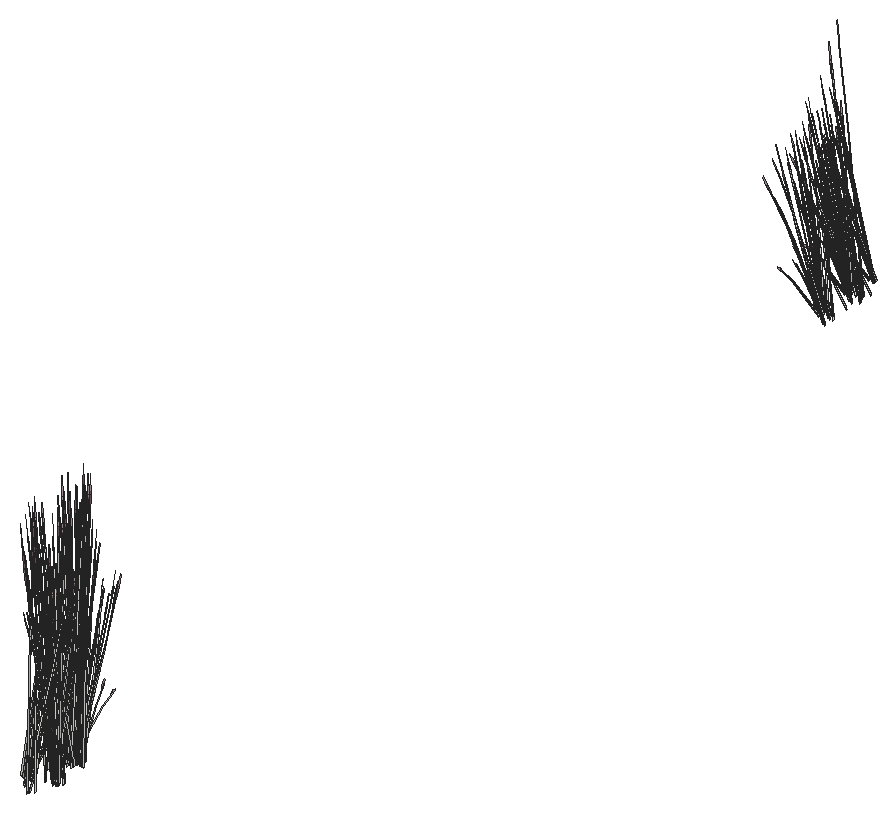
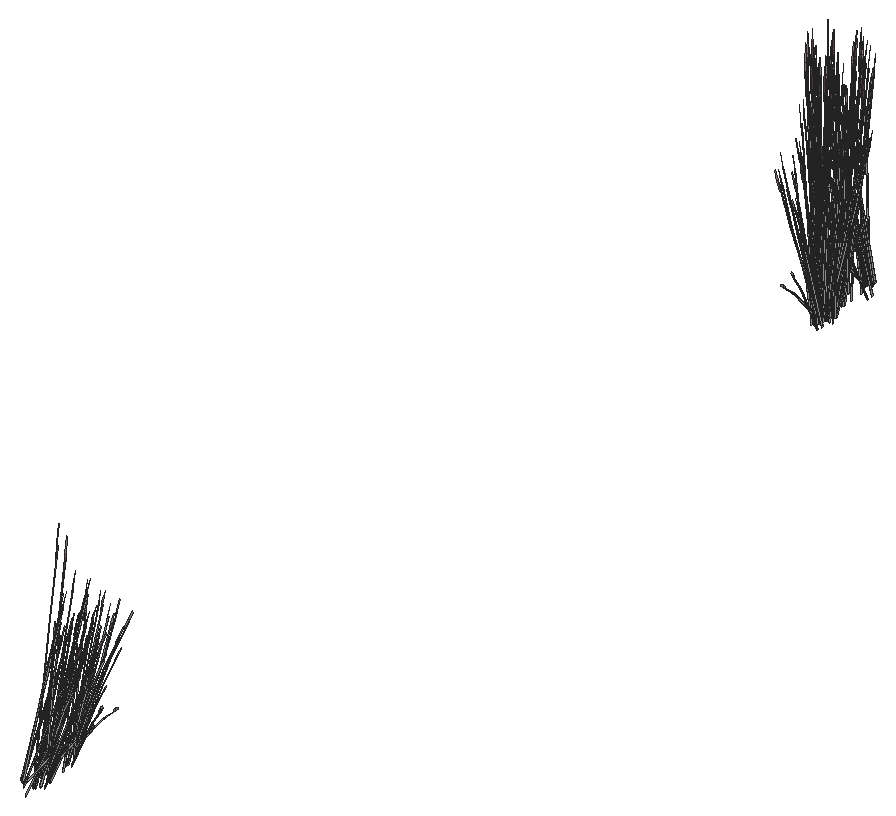
# SketchUp Ruby script. Lengths in inches.
U = 1.inch
M = Sketchup.active_model
def pt(a) = Geom::Point3d.new(a.map { |v| v * U })
def face(e, loops, mat)
  f = e.add_face(loops[0].map { |a| pt(a) })
  loops[1..].each { |l| e.add_face(l.map { |a| pt(a) }).erase! }
  f.material = f.back_material = mat if mat
  f
end
# faces: each face lists its corners as indices into pts; further lists are holes
def faces(e, pts, list, mat = nil) = list.each { |f| face(e, (f[0].is_a?(Array) ? f : [f]).map { |l| l.map { |i| pts[i] } }, mat) }
# xy, xz, yz: faces in a plane at the given z, y or x. An outline is a flat list of corners, or four numbers for a rectangle; further outlines are holes
def ring(l) = l.size == 4 ? [[l[0], l[1]], [l[2], l[1]], [l[2], l[3]], [l[0], l[3]]] : l.each_slice(2).to_a
def flat(e, list, mat, &to3) = list.each { |f| face(e, (f[0].is_a?(Array) ? f : [f]).map { |l| ring(l).map { |u, v| to3.(u, v) } }, mat) }
def xy(e, z, list, mat = nil) = flat(e, list, mat) { |x, y| [x, y, z] }
def xz(e, y, list, mat = nil) = flat(e, list, mat) { |x, z| [x, y, z] }
def yz(e, x, list, mat = nil) = flat(e, list, mat) { |y, z| [x, y, z] }
def lines(e, pts, list) = list.each { |a, b| e.add_line(pt(pts[a]), pt(pts[b])) }
# prism: a flat outline (further loops are holes) pulled along v
def prism(e, loops, v, mat = nil)
  f = face(e, loops, mat); d = Geom::Vector3d.new(v.map { |x| x * U })
  f.pushpull(f.normal.samedirection?(d) ? d.length : -d.length)
end
def box(e, o, s, mat = nil) = prism(e, [[o, [o[0] + s[0], o[1], o[2]], [o[0] + s[0], o[1] + s[1], o[2]], [o[0], o[1] + s[1], o[2]]]], [0, 0, s[2]], mat)
def at(x, y, z, deg = 0) = Geom::Transformation.translation(pt([x, y, z])) * Geom::Transformation.rotation(ORIGIN, Z_AXIS, deg.degrees)
def axes(o, x, y, z) = Geom::Transformation.new([*x, 0, *y, 0, *z, 0, *pt(o).to_a, 1])
def part(name) = M.definitions.add(name)
# library, detail: a bought-in or finely detailed component or shape, given as its bounding box
def library(name, o, s) = part(name).tap { |d| box(d.entities, o, s) }
def detail(e, o, s) = box(e.add_group.entities, o, s)
def put(e, d, t, mat = nil) = e.add_instance(d, t).tap { |i| i.material = mat if mat }
def group(e, t, mat = nil) = e.add_group.tap { |g| g.transformation = t; g.material = mat if mat }.entities
root = M.entities
M.materials.add("LightPink_Translucent").color = [144, 107, 117]
M.materials["LightPink_Translucent"].alpha = 0.75
c1 = part("blade")
p = [[2.15,0.21,22],[0,0.17,0],[0.09,0.45,0],[2.18,0.31,22],[2.29,0.31,22],[0.38,0.45,0],
  [2.48,0.24,33],[2.49,0.24,33],[2.48,0.22,33]]
faces(c1.entities,p,[[0,1,2,3],[4,5,2,3],[6,3,4,7],[8,0,3,6]])
c2 = part("seeds")
p = [[0.3,-0.1,1.38],[-0.01,-0.03,1.59],[-0.01,-0.03,0.03],[0.14,-0.07,-0.07],[0.29,-0.03,3],[0.15,0.01,3.11]]
faces(c2.entities,p,[[0,1,2,3],[1,0,4,5]],"LightPink_Translucent")
c3 = part("blade with seeds")
put(c3.entities,c1,at(0,0,0))
put(c3.entities,c2,axes([2.4,0.25,30.99],[1.5799,-0.05474,1.17369],[-0.12525,1.92788,0.29478],[-0.07173,-0.02425,1.56792]))
put(root,c3,axes([406.86,60.78,-9.79],[0.31974,0.54466,0],[-0.53494,0.30375,-0.48057],[-0.12184,0.06918,1.52448]))
put(root,c3,axes([406.59,58.62,-9.35],[-0.01397,-0.51177,1.31553],[0.63227,0.13266,0.557],[-0.14954,0.28003,1.24175]))
put(root,c3,axes([405.24,60.67,-7.3],[0.15418,-0.41799,0.32977],[0.44981,0.12192,-0.42575],[0.04124,0.16829,0.81462]))
put(root,c3,axes([406.28,64.63,-9.69],[0,0.54355,0.46235],[-0.57217,0,0],[0,-0.1238,1.46668]))
put(root,c3,axes([407.63,65.07,-9.94],[-0.30722,-0.45622,-0.41661],[0.46535,-0.32126,0.2005],[-0.09942,-0.05645,1.33761]))
put(root,c3,axes([407.58,64.91,-9.47],[-0.24813,0.48978,0.41661],[-0.51557,-0.23571,-0.2005],[0,-0.1129,1.33761]))
put(root,c3,axes([405.85,62.16,-6.74],[0.35341,-0.31182,-0.06041],[0.32382,0.34152,-0.27392],[0.0228,0.09677,0.90349]))
put(root,c3,axes([405.1,61.05,-7.6],[-0.37684,0.18473,0.05988],[-0.18445,-0.33686,0.47138],[0.03639,0.14849,0.71878]))
put(root,c3,axes([404.05,60.28,-6.97],[0.56206,0.02693,-0.12569],[-0.01536,0.50991,-0.69765],[-0.03904,0.19638,1.06006]))
put(root,c3,axes([405.09,60.84,-7.3125],[0.50045,-0.25306,-0.11324],[0.24593,0.44915,-0.62851],[0.06603,0.18927,0.95501]))
put(root,c3,axes([405.24,61.01,-7.28],[-0.50393,-0.1421,0.49617],[0.17232,-0.46717,0.40911],[0.03028,0.18372,1.0267]))
put(root,c3,axes([407.75,65.02,-9.8],[0.64638,0.11452,0.42607],[-0.13155,0.64678,0.16719],[-0.09446,-0.06245,1.47927]))
put(root,c3,axes([405.18,60.94,-10.61],[0.08277,-0.02958,1.6421],[0.49786,0.16279,-0.25086],[0.01456,0.18348,0.2797]))
put(root,c3,axes([406.79,66.08,-10.11],[-0.12013,-0.47362,-0.28847],[0.47712,-0.13449,0.28847],[-0.09619,-0.05462,1.29413]))
put(root,c3,axes([404.4375,60.47,-7.34],[0.3661,0.36521,-0.52818],[-0.38674,0.31985,-0.40911],[-0.0557,0.18556,1.01061]))
put(root,c3,axes([404.04,61.02,-9.37],[0.46459,-0.09625,0.0606],[0.10681,0.38778,-0.80367],[-0.02945,0.1963,0.72038]))
put(root,c3,axes([405.52,60.82,-7.64],[0.50273,0.13626,-0.47583],[-0.17232,0.46717,-0.36857],[0.0461,0.18809,0.91046]))
put(root,c3,axes([406.65,66.29,-10.12],[-0.47863,-0.27177,-0.46235],[0.28609,-0.48733,0],[-0.10901,-0.0619,1.46668]))
put(root,c3,axes([405.29,61.11,-7.78],[-0.15418,0.41799,-0.32977],[-0.44981,-0.12192,0.42575],[0.04124,0.16829,0.81462]))
put(root,c3,axes([407.95,65.33,-9.52],[-0.51635,0.36087,-0.27094],[-0.34336,-0.5099,-0.46562],[-0.1274,-0.05178,1.4872]))
put(root,c3,axes([404.85,59.94,-8.39],[-0.01252,-0.20862,1.59586],[0.54251,0.1384,0.12904],[-0.03356,0.2973,0.68222]))
put(root,c3,axes([407.91,65.49,-9.5625],[-0.09866,0.48509,0.13483],[-0.48202,-0.0842,-0.38503],[-0.08772,-0.04981,1.18024]))
put(root,c3,axes([405.34,60.73,-7.36],[0.24409,0.44196,-0.66157],[-0.50245,0.2463,0.07984],[0.05708,0.21354,0.93586]))
put(root,c3,axes([404.97,61.85,-7.61],[0.06483,0.08753,1.62908],[0.52315,0.03439,-0.25764],[0.05261,0.19303,0.13065]))
put(root,c3,axes([408.53,65.49,-9.7],[-0.49938,-0.43748,-0.23459],[0.42021,-0.49126,0.51337],[-0.13447,0.05118,1.56642]))
put(root,c3,axes([407.22,66.33,-9.69],[0.47863,0.27177,0.46235],[-0.28609,0.48733,0],[-0.10901,-0.0619,1.46668]))
put(root,c3,axes([406.94,66.61,-9.79],[-0.31974,0.54466,0],[-0.53494,-0.30375,-0.48057],[-0.12184,-0.06918,1.52448]))
put(root,c3,axes([405.96,70.8125,-7.36],[-0.24409,-0.44196,-0.66157],[0.50245,-0.2463,0.07984],[-0.05708,-0.21354,0.93586]))
put(root,c3,axes([408.28,65.4,-9.94],[-0.55535,0.03355,-0.41661],[-0.05022,-0.55698,0.2005],[-0.09942,0.05645,1.33761]))
put(root,c3,axes([405.54,69.83,-10.61],[-0.08578,0.01958,1.6421],[-0.47437,-0.22044,-0.25086],[0.00796,-0.18387,0.2797]))
put(root,c3,axes([408.9,66.69,-9.96],[-0.31576,-0.54657,-0.04789],[0.53494,-0.30375,0.48057],[-0.13182,0.05204,1.52373]))
put(root,c3,axes([406,70.4375,-7.78],[0.15418,-0.41799,-0.32977],[0.44981,0.12192,0.42575],[-0.04124,-0.16829,0.81462]))
put(root,c3,axes([407.64,70.07,-7.62],[-0.05194,0.04152,1.65179],[-0.50886,-0.14007,-0.15608],[-0.01842,-0.18118,0.29231]))
put(root,c3,axes([405.77,70.73,-7.64],[-0.50273,-0.13626,-0.47583],[0.17232,-0.46717,-0.36857],[-0.0461,-0.18809,0.91046]))
put(root,c3,axes([406.08,69.56,-9.42],[0.06561,0.31695,1.06958],[-0.36394,-0.17555,0.78586],[0.03916,-0.16229,0.23558]))
put(root,c3,axes([408.75,66.62,-10.11],[-0.47712,-0.13449,-0.28847],[0.12013,-0.47362,0.28847],[-0.09619,0.05462,1.29413]))
put(root,c3,axes([406.11,65.29,-7.3],[0.44516,-0.07768,0.32977],[0.11755,0.44407,-0.42575],[-0.12757,0.11927,0.81462]))
put(root,c3,axes([406.06,70.54,-7.59],[0.50393,0.1421,0.447],[-0.17232,0.46717,0.36857],[-0.03028,-0.18372,0.92496]))
put(root,c3,axes([406.2,70.7,-7.3125],[-0.50045,0.25306,-0.11324],[-0.24593,-0.44915,-0.62851],[-0.06603,-0.18927,0.95501]))
put(root,c3,axes([407.24,71.27,-7.3125],[-0.56206,-0.02693,-0.11324],[0.01536,-0.50991,-0.62851],[0.03904,-0.19638,0.95501]))
put(root,c3,axes([406.19,70.5,-7.6],[0.37684,-0.18473,0.05988],[0.18445,0.33686,0.47138],[-0.03639,-0.14849,0.71878]))
put(root,c3,axes([408.67,65.25,-9.52],[0.05959,0.62022,-0.27094],[-0.62068,0.0375,-0.46562],[-0.1093,0.08261,1.4872]))
put(root,c3,axes([405.1,66.55,-6.74],[0.45129,0.14509,-0.06041],[-0.13882,0.44656,-0.27392],[-0.07381,0.0678,0.90349]))
put(root,c3,axes([408.3,65.72,-10.08],[-0.34446,0.40855,-0.58063],[-0.42791,-0.37046,-0.15239],[-0.13803,0.10191,1.28164]))
put(root,c3,axes([404.83,72.47,-10.05],[-0.21003,-0.55738,-0.65031],[0.60499,-0.20074,-0.17068],[-0.02321,-0.18874,1.43544]))
put(root,c3,axes([408.86,66.84,-10.12],[-0.47863,0.27177,-0.46235],[-0.28609,-0.48733,0],[-0.10901,0.0619,1.46668]))
put(root,c3,axes([406.05,70.88,-7.3],[-0.15418,0.41799,0.32977],[-0.44981,-0.12192,-0.42575],[-0.04124,-0.16829,0.81462]))
put(root,c3,axes([405.875,65.25,-7.3125],[0.47307,0.29971,-0.11324],[-0.27254,0.43404,-0.62851],[-0.13365,0.15087,0.95501]))
put(root,c3,axes([404.75,70.87,-9.79],[-0.31974,-0.54466,0],[0.53494,-0.30375,-0.48057],[0.12184,-0.06918,1.52448]))
put(root,c3,axes([406.71,66.17,-7.3],[0.34603,-0.28618,0.32977],[0.32756,0.32677,-0.42575],[-0.04984,0.16603,0.81462]))
put(root,c3,axes([405.45,70.22,-10.02],[-0.35341,0.31182,-0.03625],[-0.32382,-0.34152,-0.16435],[-0.0228,-0.09677,0.54209]))
put(root,c3,axes([409.03,64.6,-9.35],[-0.01397,-0.51177,1.31553],[0.63227,0.13266,0.557],[-0.14954,0.28003,1.24175]))
put(root,c3,axes([406.39,66.43,-7.6],[-0.42027,-0.02533,0.05988],[0.01152,-0.38243,0.47138],[-0.04398,0.14649,0.71878]))
put(root,c3,axes([406.53,66.47,-7.59],[-0.36417,-0.37086,0.447],[0.38674,-0.31985,0.36857],[-0.06718,0.174,0.92496]))
put(root,c3,axes([405.15,72.62,-9.94],[0.24813,-0.48978,-0.41661],[0.51557,0.23571,0.2005],[0,-0.1129,1.33761]))
put(root,c3,axes([406.53,66.58,-7.78],[-0.34603,0.28618,-0.32977],[-0.32756,-0.32677,0.42575],[-0.04984,0.16603,0.81462]))
put(root,c3,axes([406.49,66.25,-6.97],[0.56206,0.02693,-0.12569],[-0.01536,0.50991,-0.69765],[-0.03904,0.19638,1.06006]))
put(root,c3,axes([403.84,72.41,-10.11],[0.35699,-0.33913,-0.28847],[0.35699,0.33913,0.28847],[0,-0.10923,1.29413]))
put(root,c3,axes([406.75,67.69,-9.42],[-0.01324,-0.32319,1.06958],[0.33072,0.23052,0.78586],[-0.06504,0.15405,0.23558]))
put(root,c3,axes([405.09,73.03,-9.52],[-0.57594,-0.25935,-0.27094],[0.27732,-0.5474,-0.46562],[-0.0181,-0.1344,1.4872]))
put(root,c3,axes([406.87,66.44,-7.34],[0.3661,0.36521,-0.52818],[-0.38674,0.31985,-0.40911],[-0.0557,0.18556,1.01061]))
put(root,c3,axes([406.47,66.99,-9.37],[0.46459,-0.09625,0.0606],[0.10681,0.38778,-0.80367],[-0.02945,0.1963,0.72038]))
put(root,c3,axes([406.76,66.28,-7.03],[-0.01331,0.50278,-0.73435],[-0.56035,-0.03377,0.08862],[-0.05914,0.213,1.03881]))
put(root,c3,axes([405.29,67.6,-7.62],[0.05802,-0.03282,1.65179],[0.47954,0.21828,-0.15608],[-0.01127,0.18175,0.29231]))
put(root,c3,axes([407.29,65.92,-8.39],[-0.01252,-0.20862,1.59586],[0.54251,0.1384,0.12904],[-0.03356,0.2973,0.68222]))
put(root,c3,axes([405.46,72.86,-9.73],[0.57623,0.26344,0.22409],[-0.27732,0.5474,0.46562],[0,-0.12618,1.49497]))
put(root,c3,axes([406.36,67.4,-9.59],[0.16138,-0.08575,1.33163],[0.39845,0.25854,-0.28638],[-0.1186,0.22371,0.56934]))
put(root,c3,axes([405.27,72.49,-9.47],[-0.55535,0.03355,0.41661],[-0.05022,-0.55698,-0.2005],[0.09942,-0.05645,1.33761]))
put(root,c3,axes([405.25,72.7,-9.8],[0.22235,0.6078,0.42607],[-0.63531,0.21135,0.16719],[0.00776,-0.11168,1.47927]))
put(root,c3,axes([405.14,73.17,-9.47],[-0.24813,0.48978,0.41661],[-0.51557,-0.23571,-0.2005],[0,-0.1129,1.33761]))
put(root,c3,axes([406.05,72.75,-9.95],[0,-0.62892,0],[0.63949,0,0],[0,0,1.6711]))
put(root,c3,axes([406.57,66.98,-8.87],[0.01124,-0.2806,1.43727],[0.50537,0.14821,0.19862],[-0.04379,0.29905,0.67868]))
put(root,c3,axes([405.75,72.35,-9.8],[-0.42403,0.49328,0.42607],[-0.50377,-0.43543,0.16719],[0.10223,-0.04923,1.47927]))
put(root,c3,axes([406.21,73.23,-9.86],[-0.47569,-0.46784,-0.05709],[0.47598,-0.46812,0],[-0.01661,-0.01634,1.63492]))
put(root,c3,axes([405.01,71.54,-9.7],[-0.14774,0.54019,0.16428],[-0.54062,-0.15287,0.32672],[0.09339,-0.00263,1.49371]))
put(root,c3,axes([405.31,73.29,-9.8],[0.64638,0.11452,0.42607],[-0.13155,0.64678,0.16719],[-0.09446,-0.06245,1.47927]))
put(root,c3,axes([404.96,74.32,-9.7],[0.54955,-0.14427,0.16428],[0.1357,0.53689,0.32672],[-0.04901,-0.07823,1.49371]))
put(root,c3,axes([406.65,71.57,-9.7],[-0.54955,0.14427,0.16428],[-0.1357,-0.53689,0.32672],[0.04901,0.07823,1.49371]))
put(root,c3,axes([406.3,72.6,-9.78],[-0.64638,-0.11452,0.45814],[0.13155,-0.64678,0.17978],[0.09446,0.06245,1.59061]))
put(root,c3,axes([405.78,74.2,-9.95],[-0.16686,-0.46861,0],[0.47648,-0.16411,0],[0,0,1.4375]))
put(root,c3,axes([406.59,74.35,-9.7],[0.14774,-0.54019,0.16428],[0.54062,0.15287,0.32672],[-0.09339,0.00263,1.49371]))
put(root,c3,axes([406.47,73.13,-9.9375],[0.35699,0.35109,0],[-0.35699,0.35109,0],[0,0,1.57621]))
put(root,c3,axes([407.4375,72.98,-9.7],[-0.40181,-0.39593,0.16428],[0.40492,-0.38402,0.32672],[-0.04438,0.08086,1.49371]))
put(root,c3,axes([405.67,74.41,-9.95],[-0.51557,-0.24403,0],[0.24813,-0.50705,0],[0,0,1.51513]))
put(root,c3,axes([406.47,72.72,-9.47],[0.24813,-0.48978,0.41661],[0.51557,0.23571,-0.2005],[0,0.1129,1.33761]))
put(root,c3,axes([406.37,73,-9.87],[0,0.62861,-0.05249],[-0.63949,0,0],[0,0.01975,1.67027]))
put(root,c3,axes([406.33,73.4,-9.47],[0.55535,-0.03355,0.41661],[0.05022,0.55698,-0.2005],[-0.09942,0.05645,1.33761]))
put(root,c3,axes([406.25,74.42,-9.95],[0.51557,0.24403,0],[-0.24813,0.50705,0],[0,0,1.62917]))
put(root,c3,axes([406.34,73.64,-9.5625],[0.37783,0.32657,0.13483],[-0.31516,0.36844,-0.38503],[-0.08772,0.04981,1.18024]))
put(root,c3,axes([406.75,74.64,-9.69],[0.47863,-0.27177,0.46235],[0.28609,0.48733,0],[-0.10901,0.0619,1.46668]))
put(root,c3,axes([406.07,74.21,-9.87],[0.22235,0.62444,-0.05599],[-0.63531,0.21881,0],[0.00776,0.02181,1.60327]))
put(root,c3,axes([406.3125,74.89,-10.11],[-0.47712,-0.13449,-0.28847],[0.12013,-0.47362,0.28847],[-0.09619,0.05462,1.29413]))
put(root,c3,axes([407.9,73.4,-9.95],[-0.63917,-0.00435,-0.04634],[0,-0.60749,0.46507],[-0.02009,0.13829,1.47457]))
put(root,c3,axes([407.77,73.48,-10.11],[-0.35699,0.33913,-0.28847],[-0.35699,-0.33913,0.28847],[0,0.10923,1.29413]))
put(root,c3,axes([406.23,73.52,-9.52],[0.05959,0.62022,-0.27094],[-0.62068,0.0375,-0.46562],[-0.1093,0.08261,1.4872]))
put(root,c3,axes([406.46,73.27,-9.94],[-0.24813,0.48978,-0.41661],[-0.51557,-0.23571,0.2005],[0,0.1129,1.33761]))
put(root,c3,axes([406.47,74.68,-9.83],[0.64025,0.17667,0.2864],[-0.16018,0.63149,-0.33981],[-0.10597,0.07904,1.53541]))
put(root,c3,axes([404.27,74.44,-7.3],[0.34603,-0.28618,0.32977],[0.32756,0.32677,-0.42575],[-0.04984,0.16603,0.81462]))
put(root,c3,axes([406.86,75.02,-9.79],[0.31974,0.54466,0],[-0.53494,0.30375,-0.48057],[-0.12184,0.06918,1.52448]))
put(root,c3,axes([406.59,72.86,-9.35],[-0.01397,-0.51177,1.31553],[0.63227,0.13266,0.557],[-0.14954,0.28003,1.24175]))
put(root,c3,axes([405.24,74.91,-7.3],[0.15418,-0.41799,0.32977],[0.44981,0.12192,-0.42575],[0.04124,0.16829,0.81462]))
put(root,c3,axes([405.84,76.4,-6.74],[0.35341,-0.31182,-0.06041],[0.32382,0.34152,-0.27392],[0.0228,0.09677,0.90349]))
put(root,c3,axes([405.1,75.29,-7.6],[-0.37684,0.18473,0.05988],[-0.18445,-0.33686,0.47138],[0.03639,0.14849,0.71878]))
put(root,c3,axes([404.05,74.52,-6.97],[0.56206,0.02693,-0.12569],[-0.01536,0.50991,-0.69765],[-0.03904,0.19638,1.06006]))
put(root,c3,axes([405.09,75.09,-7.3125],[0.50045,-0.25306,-0.11324],[0.24593,0.44915,-0.62851],[0.06603,0.18927,0.95501]))
put(root,c3,axes([405.23,75.25,-7.28],[-0.50393,-0.1421,0.49617],[0.17232,-0.46717,0.40911],[0.03028,0.18372,1.0267]))
put(root,c3,axes([405.18,75.1875,-10.61],[0.08277,-0.02958,1.6421],[0.49786,0.16279,-0.25086],[0.01456,0.18348,0.2797]))
put(root,c3,axes([404.43,74.71,-7.34],[0.3661,0.36521,-0.52818],[-0.38674,0.31985,-0.40911],[-0.0557,0.18556,1.01061]))
put(root,c3,axes([404.03,75.26,-9.37],[0.46459,-0.09625,0.0606],[0.10681,0.38778,-0.80367],[-0.02945,0.1963,0.72038]))
put(root,c3,axes([405.52,75.07,-7.64],[0.50273,0.13626,-0.47583],[-0.17232,0.46717,-0.36857],[0.0461,0.18809,0.91046]))
put(root,c3,axes([405.29,75.35,-7.78],[-0.15418,0.41799,-0.32977],[-0.44981,-0.12192,0.42575],[0.04124,0.16829,0.81462]))
put(root,c3,axes([404.85,74.1875,-8.39],[-0.01252,-0.20862,1.59586],[0.54251,0.1384,0.12904],[-0.03356,0.2973,0.68222]))
put(root,c3,axes([405.33,74.98,-7.36],[0.24409,0.44196,-0.66157],[-0.50245,0.2463,0.07984],[0.05708,0.21354,0.93586]))
put(root,c3,axes([404.97,76.09,-7.61],[0.06483,0.08753,1.62908],[0.52315,0.03439,-0.25764],[0.05261,0.19303,0.13065]))
put(root,c3,axes([410.42,279.22,-8.39],[0.18996,0.09365,1.59586],[-0.39312,0.39287,0.12904],[-0.24502,-0.17723,0.68222]))
put(root,c3,axes([410.39,278.36,-7.61],[-0.11004,-0.00384,1.62908],[-0.35032,0.38367,-0.25764],[-0.18692,-0.07839,0.13065]))
put(root,c3,axes([410.35,279.35,-7.78],[-0.29098,-0.34031,-0.32977],[0.33226,-0.32215,0.42575],[-0.16881,-0.04902,0.81462]))
put(root,c3,axes([410.24,279.72,-9.59],[0.09985,0.15133,1.33163],[-0.23008,0.41134,-0.28638],[-0.23625,-0.09832,0.56934]))
put(root,c3,axes([410.66,279.58,-7.36],[-0.51122,-0.01309,-0.66157],[0.03434,-0.5511,0.07984],[-0.21658,-0.05816,0.93586]))
put(root,c3,axes([409.96,278.68,-7.62],[0.03791,0.05424,1.65179],[-0.18278,0.48761,-0.15608],[-0.18511,0.00353,0.29231]))
put(root,c3,axes([410.49,279.69,-7.64],[-0.37135,0.36005,-0.47583],[-0.32522,-0.38035,-0.36857],[-0.18868,-0.05478,0.91046]))
put(root,c3,axes([409.65,280.17,-9.42],[0.3265,-0.03889,1.06958],[-0.20711,0.3427,0.78586],[-0.16135,-0.05141,0.23558]))
put(root,c3,axes([410.68,279.32,-7.3125],[-0.02738,0.55277,-0.11324],[-0.51847,-0.01511,-0.62851],[-0.19968,-0.0384,0.95501]))
put(root,c3,axes([410.02,280.08,-8.39],[0.21212,-0.01231,1.59586],[-0.14072,0.53355,0.12904],[-0.3023,-0.033,0.68222]))
put(root,c3,axes([409.93,280.48,-7.59],[0.14449,-0.4956,0.447],[0.47502,0.16947,0.36857],[-0.1868,0.02978,0.92496]))
put(root,c3,axes([409.9,280.35,-7.6],[-0.18783,-0.37061,0.05988],[0.34252,-0.1814,0.47138],[-0.15099,0.03579,0.71878]))
put(root,c3,axes([409.89,280.73,-10.61],[0.01297,0.08566,1.6421],[-0.26146,0.44735,-0.25086],[-0.18572,-0.02255,0.2797]))
put(root,c3,axes([409.83,280.54,-7.78],[-0.42502,-0.15163,-0.32977],[0.12396,-0.44238,0.42575],[-0.17112,0.04056,0.81462]))
put(root,c3,axes([411.13,280.46,-8.89],[0.14537,-0.07863,1.64882],[0.05013,0.549,0.12904],[-0.31487,0.07285,0.5893]))
put(root,c3,axes([409.57,280.83,-7.61],[-0.08351,0.07057,1.62908],[0.0071,0.51561,-0.25764],[-0.19143,0.06705,0.13065]))
put(root,c3,axes([410.125,280.76,-7.64],[-0.13855,0.49442,-0.47583],[-0.47502,-0.16947,-0.36857],[-0.19125,0.04534,0.91046]))
put(root,c3,axes([410.1,280.34,-7.3125],[0.25732,0.49218,-0.11324],[-0.45669,0.24187,-0.62851],[-0.19245,0.06494,0.95501]))
put(root,c3,axes([410.11,281.02,-8.39],[0.17745,-0.11497,1.59586],[0.14939,0.53127,0.12904],[-0.27857,0.12007,0.68222]))
put(root,c3,axes([409.56,281.92,-9.59],[0.17773,0.04462,1.33163],[0.11455,0.45576,-0.28638],[-0.24142,0.08531,0.56934]))
put(root,c3,axes([408.64,281.35,-7.62],[0.06527,0.01458,1.65179],[0.20191,0.48025,-0.15608],[-0.1336,0.12605,0.29231]))
put(root,c3,axes([409.1875,282.875,-9.42],[0.21313,-0.24635,1.06958],[0.0841,0.38999,0.78586],[-0.15402,0.06983,0.23558]))
put(root,c3,axes([409.99,281.8125,-7.78],[-0.44516,0.07768,-0.32977],[-0.11755,-0.44407,0.42575],[-0.12757,0.11927,0.81462]))
put(root,c3,axes([410.14,288.19,-7.36],[-0.43608,-0.26272,-0.66157],[0.30991,-0.46038,0.07984],[-0.158,-0.15687,0.93586]))
put(root,c3,axes([410.76,281.375,-8.39],[0.12773,-0.16701,1.59586],[0.32252,0.4508,0.12904],[-0.22121,0.20529,0.68222]))
put(root,c3,axes([409.75,283.13,-10.61],[0.0686,0.0543,1.6421],[0.11632,0.50315,-0.25086],[-0.15204,0.10729,0.2797]))
put(root,c3,axes([409.29,287.76,-10.61],[-0.04954,0.0716,1.6421],[-0.50062,0.15438,-0.25086],[-0.12094,-0.14044,0.2797]))
put(root,c3,axes([409.02,288.48,-8.39],[0.18996,0.09365,1.59586],[-0.39312,0.39287,0.12904],[-0.24502,-0.17723,0.68222]))
put(root,c3,axes([409.9375,288.21,-7.64],[-0.50465,0.12921,-0.47583],[-0.08828,-0.48932,-0.36857],[-0.13555,-0.14022,0.91046]))
put(root,c3,axes([410.29,287.77,-6.94],[-0.34131,0.52108,-0.12682],[-0.49429,-0.3002,-0.70393],[-0.17182,-0.14722,1.06961]))
put(root,c3,axes([408.98,287.62,-7.61],[-0.11004,-0.00384,1.62908],[-0.35032,0.38367,-0.25764],[-0.18692,-0.07839,0.13065]))
put(root,c3,axes([408.9,288.49,-7.26],[0.42234,-0.40113,0.50064],[0.36424,0.42599,0.4128],[-0.19815,-0.07399,1.03595]))
put(root,c3,axes([409.09,288.48,-7.6],[0.02575,-0.41332,0.05988],[0.38885,0.01133,0.47138],[-0.14895,-0.04325,0.71878]))
put(root,c3,axes([408.95,288.62,-7.78],[-0.29098,-0.34031,-0.32977],[0.33226,-0.32215,0.42575],[-0.16881,-0.04902,0.81462]))
put(root,c3,axes([408.84,288.98,-9.59],[0.09985,0.15133,1.33163],[-0.23008,0.41134,-0.28638],[-0.23625,-0.09832,0.56934]))
put(root,c3,axes([409.25,288.84,-7.36],[-0.51122,-0.01309,-0.66157],[0.03434,-0.5511,0.07984],[-0.21658,-0.05816,0.93586]))
put(root,c3,axes([408.56,287.94,-7.62],[0.03791,0.05424,1.65179],[-0.18278,0.48761,-0.15608],[-0.18511,0.00353,0.29231]))
put(root,c3,axes([409.08,288.95,-7.64],[-0.37135,0.36005,-0.47583],[-0.32522,-0.38035,-0.36857],[-0.18868,-0.05478,0.91046]))
put(root,c3,axes([409.36,288.79,-7.3],[0.29098,0.34031,0.32977],[-0.33226,0.32215,-0.42575],[-0.16881,-0.04902,0.81462]))
put(root,c3,axes([408.25,289.43,-9.42],[0.3265,-0.03889,1.06958],[-0.20711,0.3427,0.78586],[-0.16135,-0.05141,0.23558]))
put(root,c3,axes([409.28,288.58,-7.3125],[-0.02738,0.55277,-0.11324],[-0.51847,-0.01511,-0.62851],[-0.19968,-0.0384,0.95501]))
put(root,c3,axes([410.2,290.77,-10.08],[-0.53199,-0.08911,-0.58063],[0.11226,-0.54969,-0.15239],[-0.15876,-0.06661,1.28164]))
put(root,c3,axes([408.53,289.74,-7.59],[0.14449,-0.4956,0.447],[0.47502,0.16947,0.36857],[-0.1868,0.02978,0.92496]))
put(root,c3,axes([408.49,289.61,-7.6],[-0.18783,-0.37061,0.05988],[0.34252,-0.1814,0.47138],[-0.15099,0.03579,0.71878]))
put(root,c3,axes([408.49,289.99,-10.61],[0.01297,0.08566,1.6421],[-0.26146,0.44735,-0.25086],[-0.18572,-0.02255,0.2797]))
put(root,c3,axes([409.5,291.81,-10.12],[-0.47863,-0.27177,-0.46235],[0.28609,-0.48733,0],[-0.10901,-0.0619,1.46668]))
put(root,c3,axes([408.43,289.8,-7.78],[-0.42502,-0.15163,-0.32977],[0.12396,-0.44238,0.42575],[-0.17112,0.04056,0.81462]))
put(root,c3,axes([408.88,289.75,-7.3],[0.42502,0.15163,0.32977],[-0.12396,0.44238,-0.42575],[-0.17112,0.04056,0.81462]))
put(root,c3,axes([409.73,289.72,-8.89],[0.14537,-0.07863,1.64882],[0.05013,0.549,0.12904],[-0.31487,0.07285,0.5893]))
put(root,c3,axes([410.38,294.74,-7.36],[-0.43608,-0.26272,-0.66157],[0.30991,-0.46038,0.07984],[-0.158,-0.15687,0.93586]))
put(root,c3,axes([408.16,290.09,-7.61],[-0.08351,0.07057,1.62908],[0.0071,0.51561,-0.25764],[-0.19143,0.06705,0.13065]))
put(root,c3,axes([408.72,290.02,-7.64],[-0.13855,0.49442,-0.47583],[-0.47502,-0.16947,-0.36857],[-0.19125,0.04534,0.91046]))
put(root,c3,axes([408.7,289.6,-7.3125],[0.25732,0.49218,-0.11324],[-0.45669,0.24187,-0.62851],[-0.19245,0.06494,0.95501]))
put(root,c3,axes([409.79,292.14,-9.79],[-0.31974,0.54466,0],[-0.53494,-0.30375,-0.48057],[-0.12184,-0.06918,1.52448]))
put(root,c3,axes([409.53,294.31,-10.61],[-0.04954,0.0716,1.6421],[-0.50062,0.15438,-0.25086],[-0.12094,-0.14044,0.2797]))
put(root,c3,axes([409.26,295.03,-8.39],[0.18996,0.09365,1.59586],[-0.39312,0.39287,0.12904],[-0.24502,-0.17723,0.68222]))
put(root,c3,axes([410.18,294.75,-7.64],[-0.50465,0.12921,-0.47583],[-0.08828,-0.48932,-0.36857],[-0.13555,-0.14022,0.91046]))
put(root,c3,axes([410.53,294.3125,-6.94],[-0.34131,0.52108,-0.12682],[-0.49429,-0.3002,-0.70393],[-0.17182,-0.14722,1.06961]))
put(root,c3,axes([408.65,290.98,-7.59],[-0.12683,-0.50025,0.447],[0.49754,-0.08682,0.36857],[-0.14663,0.11765,0.92496]))
put(root,c3,axes([408.55,290.88,-7.6],[-0.35109,-0.22859,0.05988],[0.2044,-0.32553,0.47138],[-0.11256,0.10524,0.71878]))
put(root,c3,axes([408.71,290.28,-8.39],[0.17745,-0.11497,1.59586],[0.14939,0.53127,0.12904],[-0.27857,0.12007,0.68222]))
put(root,c3,axes([409.22,294.16,-7.61],[-0.11004,-0.00384,1.62908],[-0.35032,0.38367,-0.25764],[-0.18692,-0.07839,0.13065]))
put(root,c3,axes([408.15,291.18,-9.59],[0.17773,0.04462,1.33163],[0.11455,0.45576,-0.28638],[-0.24142,0.08531,0.56934]))
put(root,c3,axes([407.24,290.61,-7.62],[0.06527,0.01458,1.65179],[0.20191,0.48025,-0.15608],[-0.1336,0.12605,0.29231]))
put(root,c3,axes([407.78,292.14,-9.42],[0.21313,-0.24635,1.06958],[0.0841,0.38999,0.78586],[-0.15402,0.06983,0.23558]))
put(root,c3,axes([409.14,295.03,-7.26],[0.42234,-0.40113,0.50064],[0.36424,0.42599,0.4128],[-0.19815,-0.07399,1.03595]))
